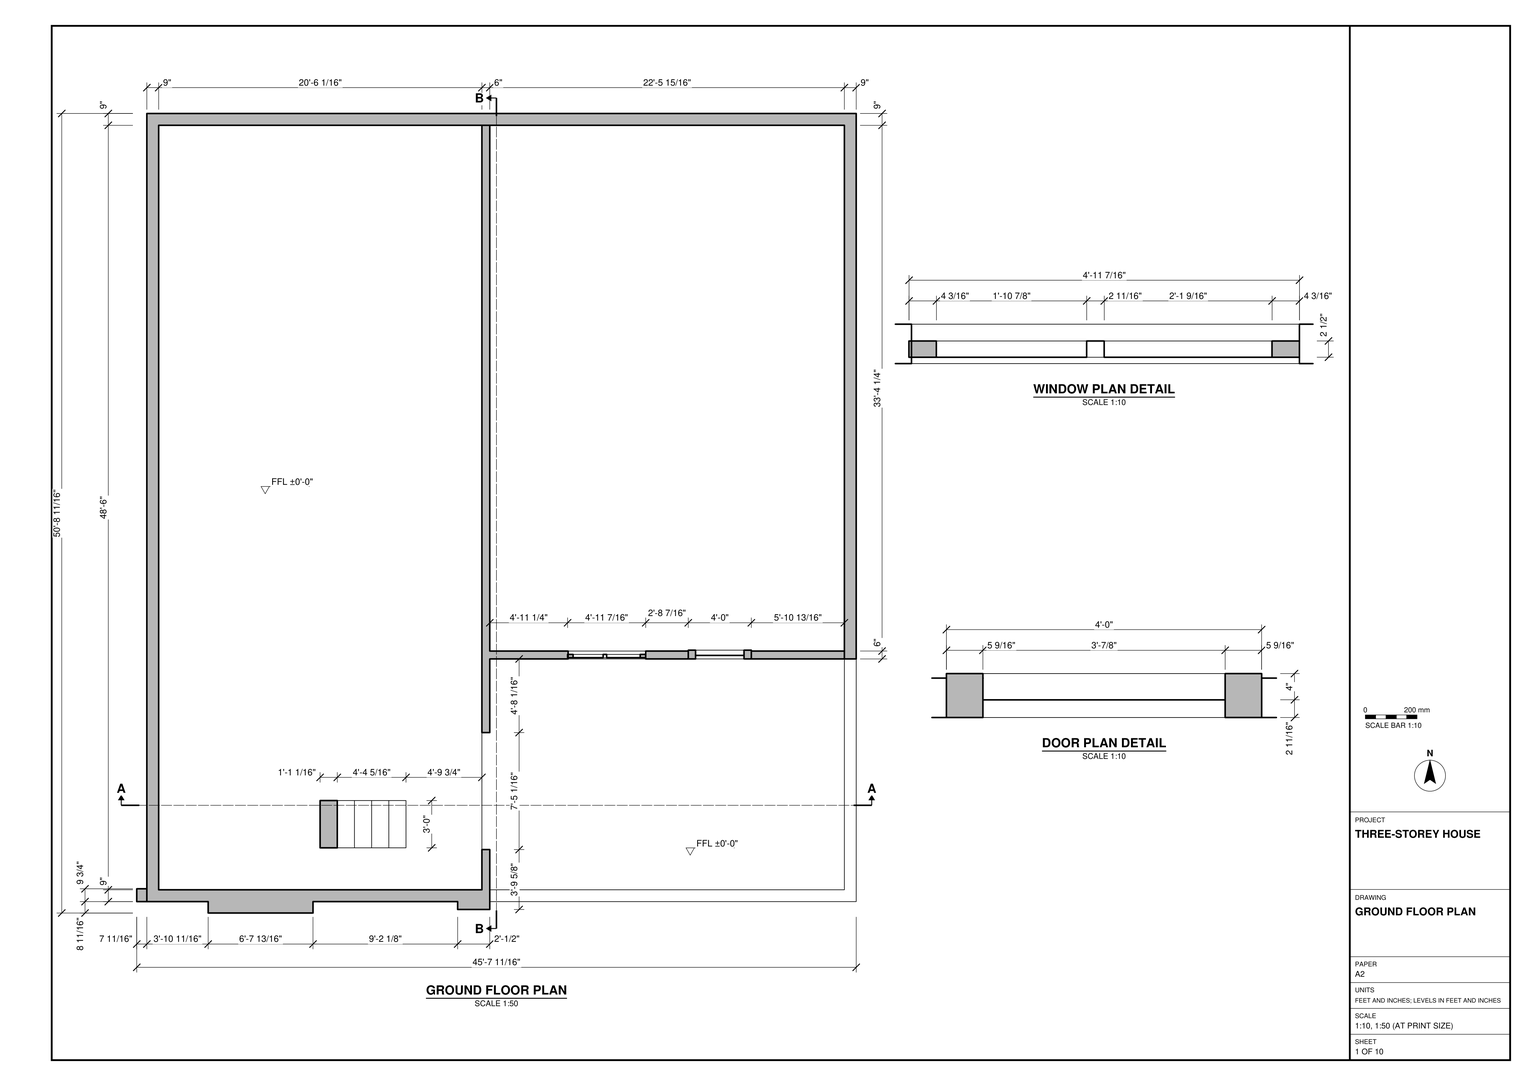
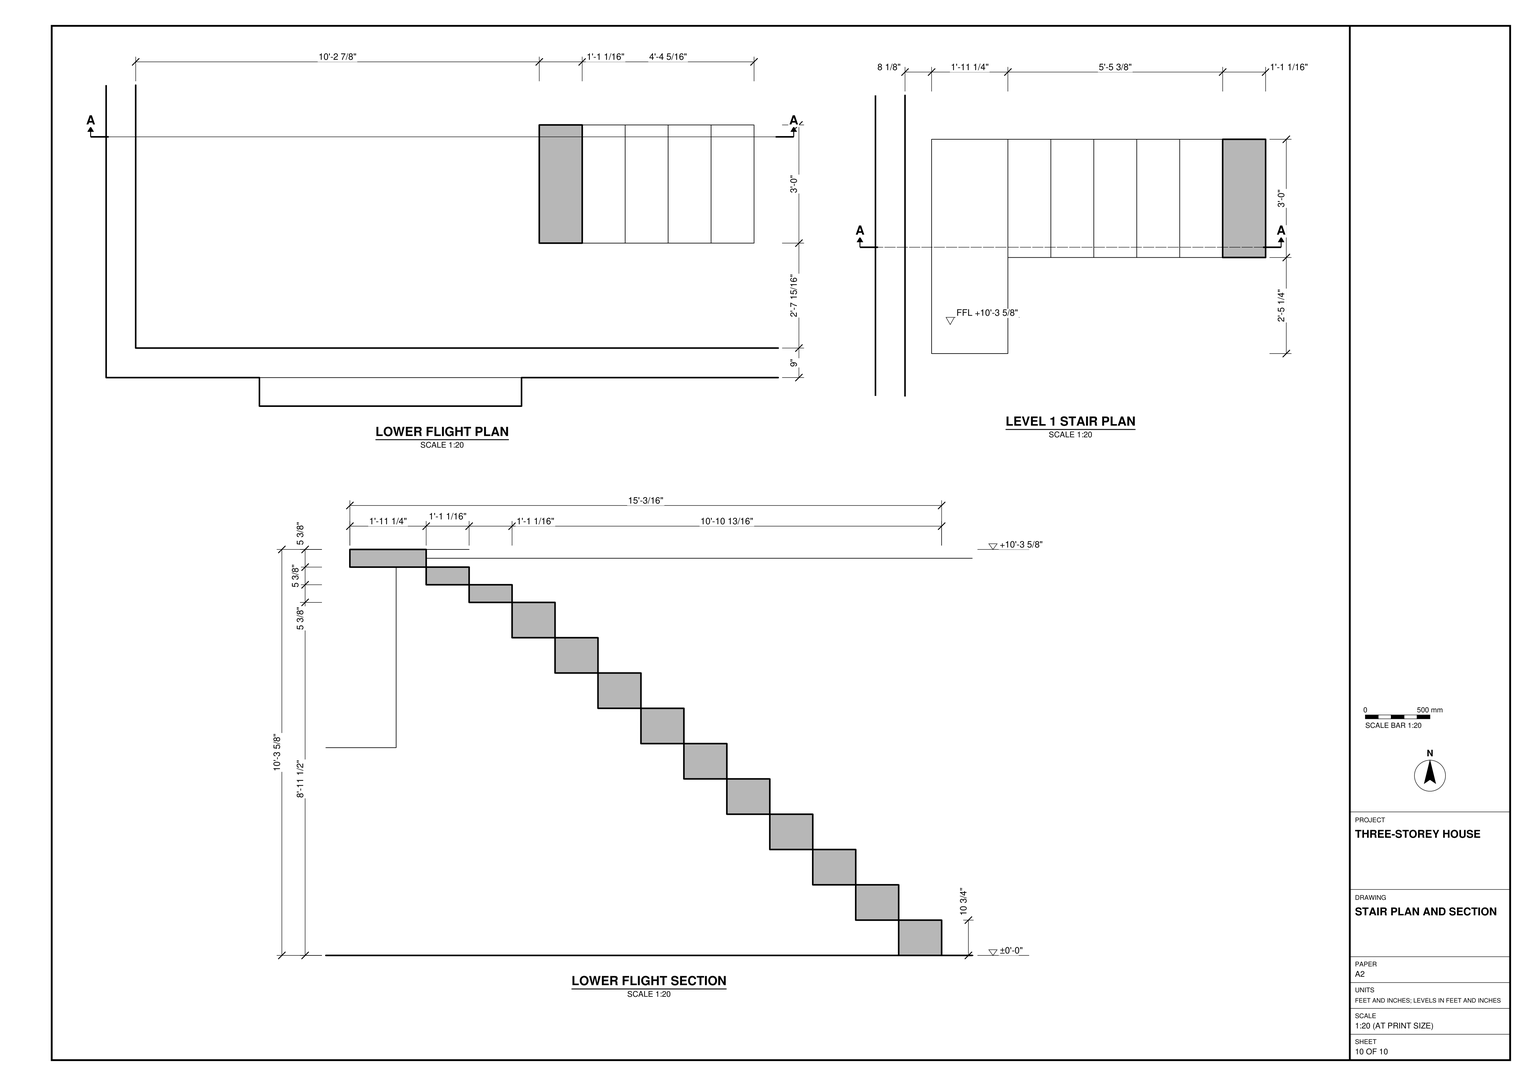
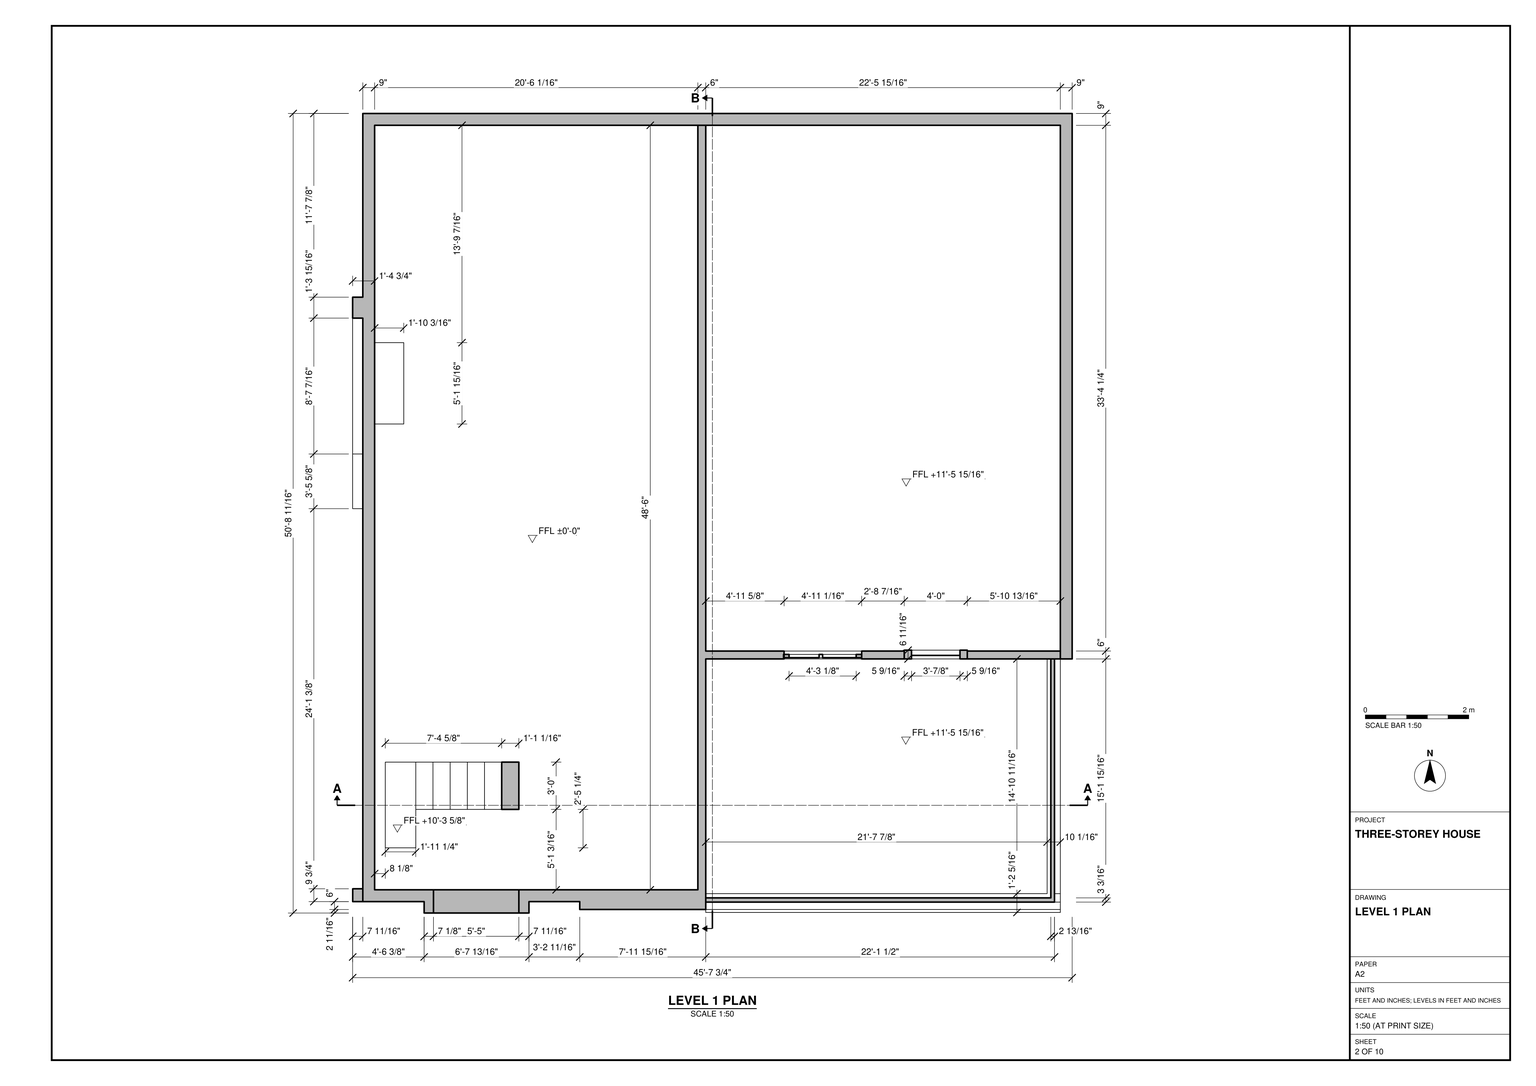
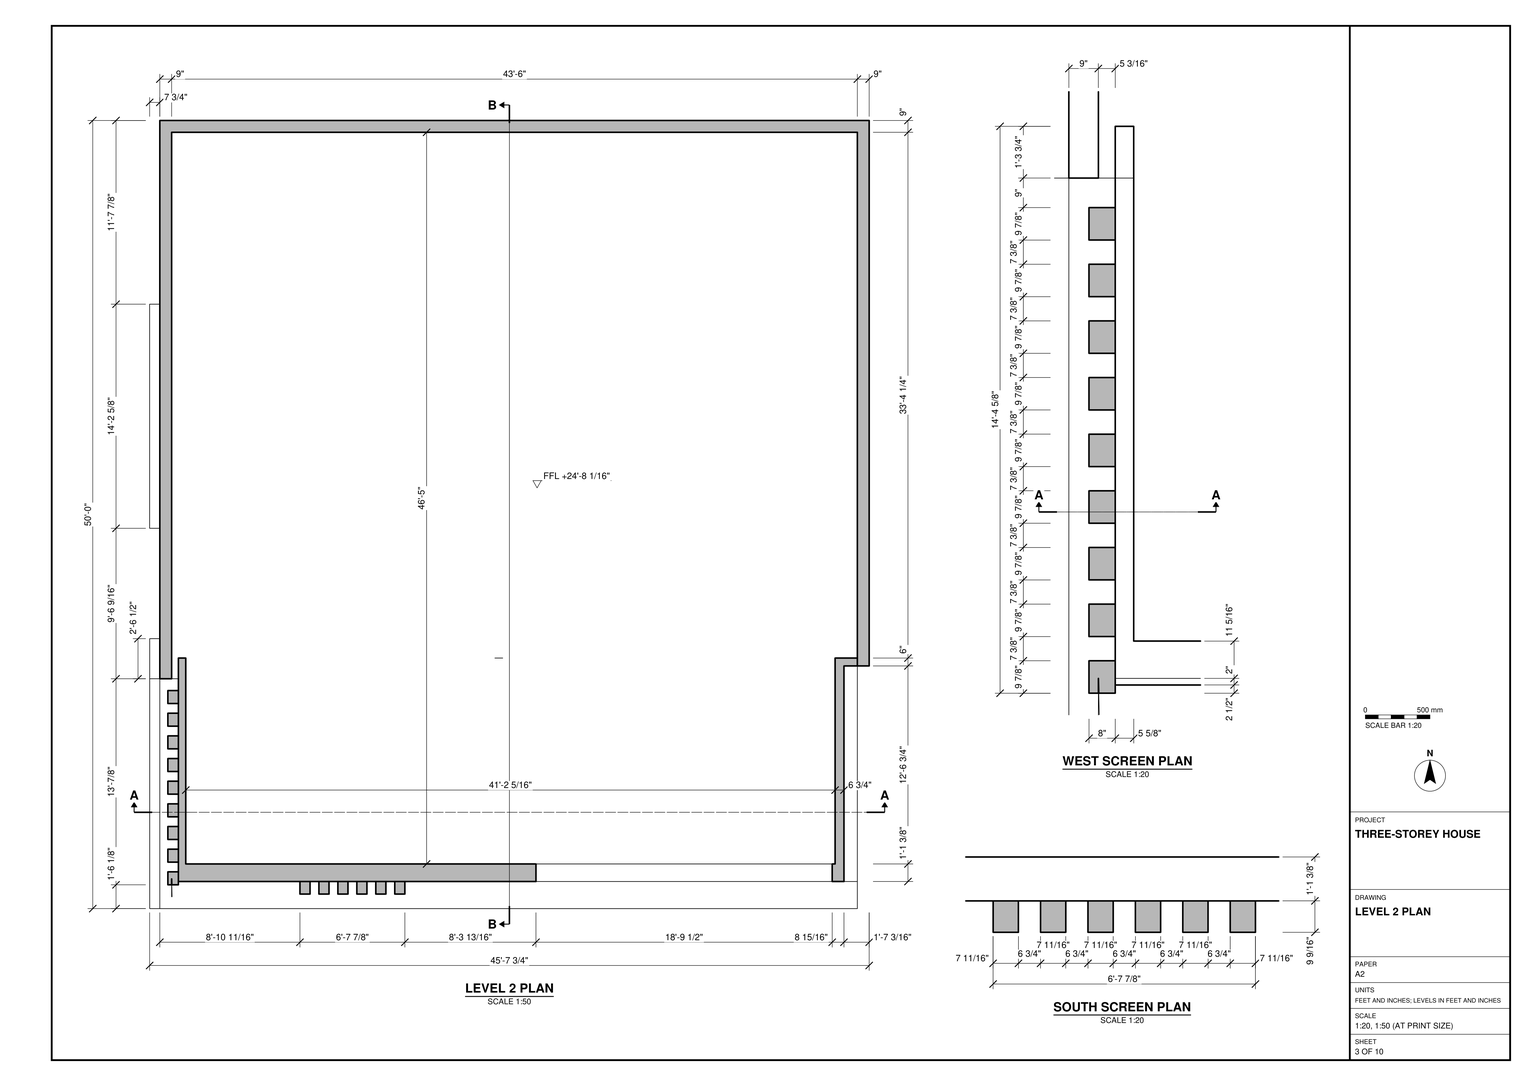
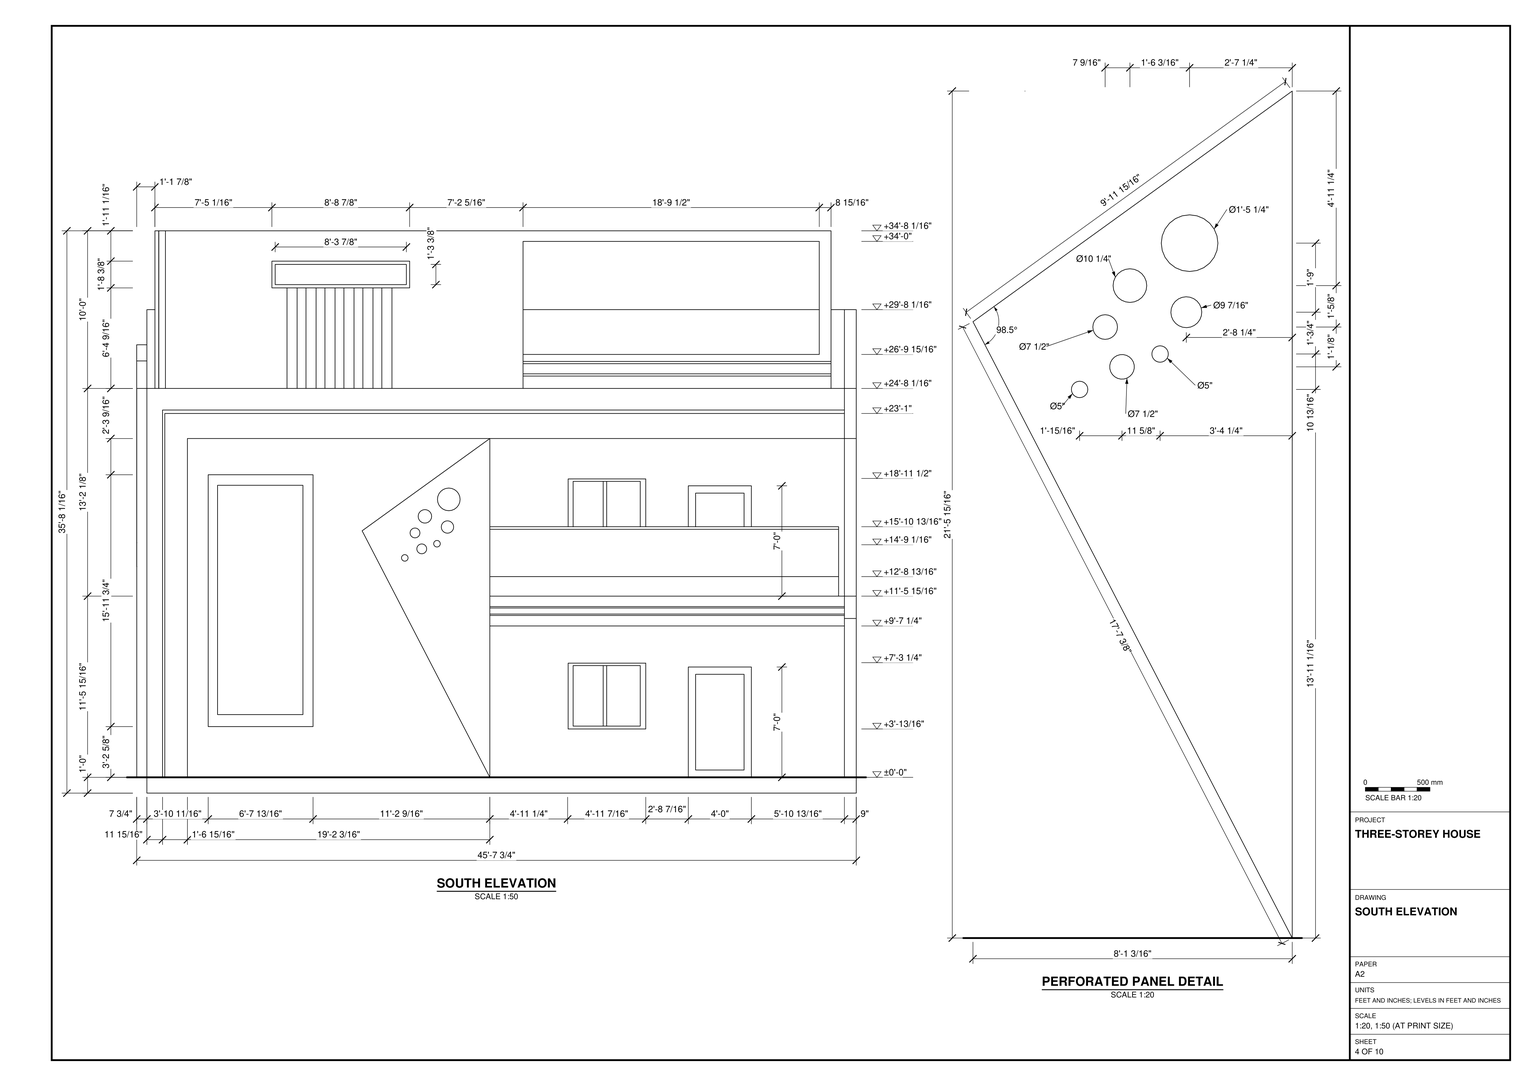
Build the three-storey house in SketchUp from task_files/diagram_01.pdf. Work in feet and inches. Set the overall width to 45'-7 3/4", depth to 50'-8 11/16" and height to 35'-8 1/16". Use finished floor levels of ±0'-0", +11'-5 15/16" and +24'-8 1/16".

Lay out the long west bay beside the wider east bay. Reproduce the wall thicknesses as dimensioned, including the 9" perimeter walls and the 6" dividing wall. Set back the south wall of the enclosed east bay and place its framed window and door according to the plan details. Model the floor slabs at their drawn extents: the Level 1 plan looks down into the west bay, while the east slab continues south beyond the recessed wall. Use the stair plans and section together to place the lower flight, form the individual steps and position the offset landing. Follow the remaining sheets for the upper storey, openings and roof profile. Include built-in joinery and main furniture where shown.

Keep walls, slabs and roof elements in separate groups or components. Group each furniture or joinery piece separately and use components for repeated parts. Any decor or loose items shown may use suitable library components. Save one SketchUp model as output_files/three_storey_house_with_a_recessed_east_bay.skp.

# SketchUp Ruby script. Lengths in inches.
U = 1.inch
M = Sketchup.active_model
def pt(a) = Geom::Point3d.new(a.map { |v| v * U })
def face(e, loops, mat)
  f = e.add_face(loops[0].map { |a| pt(a) })
  loops[1..].each { |l| e.add_face(l.map { |a| pt(a) }).erase! }
  f.material = f.back_material = mat if mat
  f
end
# faces: each face lists its corners as indices into pts; further lists are holes
def faces(e, pts, list, mat = nil) = list.each { |f| face(e, (f[0].is_a?(Array) ? f : [f]).map { |l| l.map { |i| pts[i] } }, mat) }
# xy, xz, yz: faces in a plane at the given z, y or x. An outline is a flat list of corners, or four numbers for a rectangle; further outlines are holes
def ring(l) = l.size == 4 ? [[l[0], l[1]], [l[2], l[1]], [l[2], l[3]], [l[0], l[3]]] : l.each_slice(2).to_a
def flat(e, list, mat, &to3) = list.each { |f| face(e, (f[0].is_a?(Array) ? f : [f]).map { |l| ring(l).map { |u, v| to3.(u, v) } }, mat) }
def xy(e, z, list, mat = nil) = flat(e, list, mat) { |x, y| [x, y, z] }
def xz(e, y, list, mat = nil) = flat(e, list, mat) { |x, z| [x, y, z] }
def yz(e, x, list, mat = nil) = flat(e, list, mat) { |y, z| [x, y, z] }
def lines(e, pts, list) = list.each { |a, b| e.add_line(pt(pts[a]), pt(pts[b])) }
# prism: a flat outline (further loops are holes) pulled along v
def prism(e, loops, v, mat = nil)
  f = face(e, loops, mat); d = Geom::Vector3d.new(v.map { |x| x * U })
  f.pushpull(f.normal.samedirection?(d) ? d.length : -d.length)
end
def box(e, o, s, mat = nil) = prism(e, [[o, [o[0] + s[0], o[1], o[2]], [o[0] + s[0], o[1] + s[1], o[2]], [o[0], o[1] + s[1], o[2]]]], [0, 0, s[2]], mat)
def at(x, y, z, deg = 0) = Geom::Transformation.translation(pt([x, y, z])) * Geom::Transformation.rotation(ORIGIN, Z_AXIS, deg.degrees)
def axes(o, x, y, z) = Geom::Transformation.new([*x, 0, *y, 0, *z, 0, *pt(o).to_a, 1])
def part(name) = M.definitions.add(name)
# library, detail: a bought-in or finely detailed component or shape, given as its bounding box
def library(name, o, s) = part(name).tap { |d| box(d.entities, o, s) }
def detail(e, o, s) = box(e.add_group.entities, o, s)
def put(e, d, t, mat = nil) = e.add_instance(d, t).tap { |i| i.material = mat if mat }
def group(e, t, mat = nil) = e.add_group.tap { |g| g.transformation = t; g.material = mat if mat }.entities
root = M.entities
M.materials.add("[Color A08]").color = [76, 0, 0]
M.materials.add("[Color D05]").color = [255, 191, 0]
M.materials.add("[Color D06]").color = [204, 153, 0]
M.materials.add("[Color E01]").color = [255, 255, 204]
M.materials.add("[Color M05]").color = [114, 114, 114]
M.materials.add("[Color M06]").color = [86, 86, 86]
M.materials.add("[Concrete Form 4x8]").color = [167, 170, 168]
M.materials.add("[Granite Tile]").color = [155, 148, 143]
M.materials.add("[Metal Seamed]").color = [118, 119, 115]
M.materials.add("[Pavers Flagstone Gray]").color = [162, 162, 162]
M.materials.add("[Stone Vein Gray]").color = [166, 165, 165]
M.materials.add("[Translucent Glass Blue]").color = [100, 149, 237]
M.materials["[Translucent Glass Blue]"].alpha = 0.5
M.materials.add("[Translucent Glass Gold]").color = [255, 254, 26]
M.materials["[Translucent Glass Gold]"].alpha = 0.6
M.materials.add("[Translucent Glass Gray]").color = [128, 128, 128]
M.materials["[Translucent Glass Gray]"].alpha = 0.5
c1 = part("Group\#1")
box(c1.entities,[0,0,0],[36,12,3.9375])
c2 = part("Group\#2")
box(c2.entities,[0,0,0],[36,12,3.9375])
c3 = part("Group\#4")
put(c3.entities,c1,at(12,0,82.6875,90))
put(c3.entities,c1,at(24,0,78.75,90))
g1 = group(c3.entities,at(144,0,0))
put(g1,c2,axes([-60,0,39.375],[0,1,0],[-1,0,0],[0,0,2]))
put(g1,c2,axes([-72,0,47.25],[0,1,0],[-1,0,0],[0,0,2]))
put(g1,c2,axes([-96,0,63],[0,1,0],[-1,0,0],[0,0,2]))
put(g1,c2,axes([-108,0,70.875],[0,1,0],[-1,0,0],[0,0,2]))
put(g1,c2,axes([-12,0,7.875],[0,1,0],[-1,0,0],[0,0,2]))
put(g1,c2,axes([-84,0,55.125],[0,1,0],[-1,0,0],[0,0,2]))
put(g1,c2,axes([-48,0,31.5],[0,1,0],[-1,0,0],[0,0,2]))
put(g1,c1,axes([0,0,0],[0,1,0],[-1,0,0],[0,0,2]))
put(g1,c2,axes([-24,0,15.75],[0,1,0],[-1,0,0],[0,0,2]))
put(g1,c2,axes([-36,0,23.625],[0,1,0],[-1,0,0],[0,0,2]))
c4 = part("Group\#7")
xy(c4.entities,0,[[0,0,3.44,17.08]],"[Color A08]")
xy(c4.entities,1.2,[[0,1.2,3.44,8.54],[0,8.54,3.44,9.31],[0,9.31,3.44,15.88]],"[Color A08]")
xy(c4.entities,26.4375,[[0,1.2,3.44,8.54],[0,8.54,3.44,9.31],[0,9.31,3.44,15.88]],"[Color A08]")
xy(c4.entities,27.64,[[0,0,3.44,17.08]],"[Color A08]")
xz(c4.entities,0,[[0,0,3.44,27.64]],"[Color A08]")
xz(c4.entities,1.2,[[0,1.2,3.44,26.4375]],"[Color A08]")
xz(c4.entities,8.54,[[0,1.2,3.44,26.4375]],"[Color A08]")
xz(c4.entities,9.31,[[0,1.2,3.44,26.4375]],"[Color A08]")
xz(c4.entities,15.88,[[0,1.2,3.44,26.4375]],"[Color A08]")
xz(c4.entities,17.08,[[0,0,3.44,27.64]],"[Color A08]")
yz(c4.entities,0,[[[0,0,17.08,27.64],[1.2,1.2,15.88,26.4375]]],"[Color A08]")
yz(c4.entities,0,[[1.2,1.2,8.54,26.4375],[9.31,1.2,15.88,26.4375]],"[Translucent Glass Blue]")
yz(c4.entities,3.44,[[[0,0,17.08,27.64],[1.2,1.2,15.88,26.4375]],[8.54,1.2,9.31,26.4375]],"[Color A08]")
c5 = part("Group\#8")
xy(c5.entities,0,[[0,0,48,6.6875]])
xy(c5.entities,5.56,[[5.56,0,42.44,2.6875],[5.56,2.6875,42.44,6.6875]],"[Color A08]")
xy(c5.entities,78.44,[[5.56,2.6875,42.44,6.6875]])
xy(c5.entities,78.44,[[5.56,0,42.44,2.6875]],"[Color A08]")
xy(c5.entities,84,[[0,0,48,6.6875]],"[Color A08]")
xz(c5.entities,0,[[[0,0,48,84],[5.56,5.56,42.44,78.44]]],"[Color A08]")
xz(c5.entities,2.6875,[[5.56,5.56,42.44,78.44]],"[Color A08]")
xz(c5.entities,6.6875,[[[0,0,48,84],[5.56,5.56,42.44,78.44]]],"[Color A08]")
yz(c5.entities,0,[[0,0,6.6875,84]])
yz(c5.entities,5.56,[[0,5.56,2.6875,78.44],[2.6875,5.56,6.6875,78.44]],"[Color A08]")
yz(c5.entities,42.44,[[2.6875,5.56,6.6875,78.44]])
yz(c5.entities,42.44,[[0,5.56,2.6875,78.44]],"[Color A08]")
yz(c5.entities,48,[[0,0,6.6875,84]],"[Color A08]")
xy(root,0,[[7.75,8.6875,547.75,608.6875]])
xy(root,12,[[7.75,8.6875,7.75,608.6875,547.75,608.6875,547.75,193.4375,538.75,193.4375,538.75,599.6875,16.75,599.6875,16.75,17.6875,262.8125,17.6875,262.8125,48.3125,268.8125,48.3125,268.8125,8.6875],[268.8125,8.6875,547.75,8.6875,547.75,193.4375,538.75,193.4375,538.75,17.6875,268.8125,17.6875],[16.75,17.6875,262.8125,599.6875],[262.8125,137.375,262.8125,599.6875,268.8125,599.6875,268.8125,199.4375,419.92,199.4375,419.92,193.4375,268.8125,193.4375,268.8125,137.375],[467.92,193.4375,538.75,199.4375],
  [268.8125,199.4375,538.75,599.6875]])
xy(root,12,[[0.0625,8.6875,7.75,18.46]],"[Color M05]")
xy(root,12,[[268.8125,17.6875,538.75,17.6875,538.75,193.4375,467.92,193.4375,467.92,199.4375,419.92,199.4375,419.92,193.4375,268.8125,193.4375,268.8125,137.375,262.8125,137.375,262.8125,48.3125,268.8125,48.3125]],"[Concrete Form 4x8]")
xy(root,48.8125,[[328.44,193.4375,387.5,199.4375]])
xy(root,50.625,[[54.43,0,134.24,8.6875]],"[Color M05]")
xy(root,59.76,[[61.55,0,126.55,17.6875]],"[Color M05]")
xy(root,75.27,[[7.75,372.29,38.9375,434.23]])
xy(root,96,[[419.92,193.4375,467.92,199.4375]])
xy(root,98.9375,[[328.44,193.4375,387.5,199.4375]])
xy(root,106.4,[[7.75,269.27,16.75,315.14]])
xy(root,118.63,[[61.55,6.1,126.55,13.16]],"[Color M05]")
xy(root,125.7,[[61.55,6.1,126.55,13.16]],"[Color M05]")
xy(root,127.25,[[268.8125,2.6875,538.75,193.4375]],"[Color E01]")
xy(root,132.9375,[[262.8125,48.3125,268.8125,137.375],[262.8125,137.375,262.8125,599.6875,268.8125,599.6875,268.8125,199.4375,538.75,199.4375,538.75,193.4375,268.8125,193.4375,268.8125,137.375]])
xy(root,135.24,[[268.8125,0.4375,538.75,2.6875]],"[Color D05]")
xy(root,136.3,[[268.8125,0.4375,538.75,2.6875]],"[Color D05]")
xy(root,140.92,[[268.8125,0.4375,538.75,2.6875]],"[Color D05]")
xy(root,141.99,[[268.8125,0.4375,538.75,2.6875]],"[Color D05]")
xy(root,149.9375,[[268.8125,2.6875,538.75,8.3125],[268.8125,8.3125,268.8125,14.75,528.7,14.75,528.7,193.4375,534.3125,193.4375,534.3125,8.3125],[534.3125,8.3125,538.75,14.75],[534.3125,14.75,538.75,193.4375],[419.92,193.4375,467.92,199.4375],
  [467.92,193.4375,538.75,199.4375],[268.8125,199.4375,538.75,599.6875]])
xy(root,149.9375,[[268.8125,14.75,528.7,193.4375]],"[Concrete Form 4x8]")
xy(root,162.02,[[7.75,269.27,16.75,315.14]])
xy(root,164.8125,[[268.8125,8.3125,268.8125,11.53,531.51,11.53,531.51,193.4375,534.3125,193.4375,534.3125,8.3125],[268.8125,11.53,531.51,11.53,531.51,193.4375,528.7,193.4375,528.7,14.75,268.8125,14.75]])
xy(root,165.39,[[7.75,372.29,38.9375,434.23]])
xy(root,172.42,[[0,307.84,7.75,468.84]],"[Color M06]")
xy(root,182.69,[[61.55,4.7,127.8,11.77]],"[Color M05]")
xy(root,189.0625,[[328.44,193.4375,387.5,199.4375]])
xy(root,189.75,[[61.55,4.7,127.8,11.77]],"[Color M05]")
xy(root,190.6,[[0,307.84,7.75,349.46],[0,349.46,7.75,452.89]],"[Color M06]")
xy(root,200.8125,[[268.8125,8.3125,268.8125,11.53,531.51,11.53,531.51,193.4375,534.3125,193.4375,534.3125,8.3125]])
xy(root,202.8125,[[268.8125,8.3125,534.3125,8.3125,534.3125,193.4375,531.51,193.4375,531.51,11.53,268.8125,11.53]],"[Metal Seamed]")
xy(root,204.21,[[7.75,514.29,46.5,576.23]])
xy(root,217.35,[[7.75,372.16,16.75,441.53]])
xy(root,233.9375,[[419.92,193.4375,467.92,199.4375]])
xy(root,234.33,[[61.55,0,126.55,17.6875]],"[Color M05]")
xy(root,239.1875,[[328.44,193.4375,387.5,199.4375]])
xy(root,242.375,[[54.43,0,134.24,8.6875]],"[Color M05]")
xy(root,257.21,[[7.75,269.27,187.4375,315.14]])
xy(root,269.9375,[[268.8125,8.6875,538.75,193.4375]])
xy(root,294.34,[[7.75,514.29,46.5,576.23]])
xy(root,300.5,[[0.0625,18.46,7.75,214.2]],"[Color M05]")
xy(root,302.0625,[[27.5,42.6875,27.5,183.68,16.75,183.68,16.75,599.6875,538.75,599.6875,538.75,199.4375,521.8125,199.4375,521.8125,42.6875]])
xy(root,304.27,[[7.75,269.27,187.4375,315.14]])
xy(root,308.0625,[[7.75,8.6875,538.75,8.6875,538.75,29.3125,194.3,29.3125,194.3,19.75,186.61,19.75,186.61,29.3125,179.86,29.3125,179.86,19.75,172.17,19.75,172.17,29.3125,165.42,29.3125,165.42,19.75,157.73,19.75,157.73,29.3125,150.98,29.3125,150.98,19.75,143.3,19.75,143.3,29.3125,136.55,29.3125,136.55,19.75,128.86,19.75,128.86,29.3125,122.11,29.3125,122.11,19.75,114.42,19.75,114.42,29.3125,21.875,29.3125,21.875,26.82,16.85,26.82,17.06,17.6875,16.75,17.6875,16.75,26.82,13.875,26.82,13.875,36.69,21.875,36.69,21.875,44.07,13.875,44.07,13.875,53.94,21.875,53.94,21.875,61.32,13.875,61.32,13.875,71.19,21.875,71.19,21.875,78.57,13.875,78.57,13.875,88.44,21.875,88.44,21.875,95.82,13.875,95.82,13.875,105.69,21.875,105.69,21.875,113.07,13.875,113.07,13.875,122.94,21.875,122.94,21.875,130.32,13.875,130.32,13.875,140.19,21.875,140.19,21.875,147.57,13.875,147.57,13.875,157.44,21.875,157.44,21.875,164.82,13.875,164.82,13.875,174.69,21.875,174.69,21.875,183.68,7.75,183.68],[16.75,17.6875,17.06,17.6875,16.85,26.82,16.75,26.82],[114.42,19.75,122.11,29.3125],[128.86,19.75,136.55,29.3125],[143.3,19.75,150.98,29.3125],
  [157.73,19.75,165.42,29.3125],[172.17,19.75,179.86,29.3125],[186.61,19.75,194.3,29.3125],[16.75,26.82,16.85,26.82,16.75,31.32],[21.875,29.3125,48.69,31.32],
  [48.69,29.3125,262.8125,42.6875],[262.8125,29.3125,262.8125,42.6875,521.8125,42.6875,521.8125,199.4375,538.75,199.4375,538.75,193.4375,528.5625,193.4375,528.5625,29.3125],[528.5625,29.3125,538.75,193.4375],[21.875,31.32,48.69,31.32,48.69,42.6875,27.5,42.6875,27.5,183.68,21.875,183.68],[27.5,42.6875,521.8125,42.6875,521.8125,199.4375,538.75,199.4375,538.75,599.6875,16.75,599.6875,16.75,183.68,21.875,183.68,21.875,199.4375,27.5,199.4375],
  [21.875,183.68,27.5,199.4375]])
xy(root,308.0625,[[0.0625,8.6875,7.75,183.68],[0.0625,183.68,7.75,214.2]],"[Color M05]")
xy(root,323.66,[[7.75,372.16,16.75,441.53]])
xy(root,329.01,[[0,298.21,7.75,349.46],[0,349.46,7.75,452.89]],"[Color M06]")
xy(root,333.96,[[294.1,29.3125,519.6,42.6875]])
xy(root,341.32,[[0,298.21,7.75,468.84]],"[Color M06]")
xy(root,368.0625,[[7.75,183.68,16.75,183.68,16.75,599.6875,538.75,599.6875,538.75,193.4375,547.75,193.4375,547.75,608.6875,7.75,608.6875],[528.5625,193.4375,538.75,199.4375]])
xy(root,384.62,[[114.42,25.625,122.11,29.3125],[128.86,25.625,136.55,29.3125],[143.3,25.625,150.98,29.3125],[157.73,25.625,165.42,29.3125],[172.17,25.625,179.86,29.3125],
  [186.61,25.625,194.3,29.3125]])
xy(root,384.62,[[114.42,19.75,122.11,25.625],[128.86,19.75,136.55,25.625],[143.3,19.75,150.98,25.625],[157.73,19.75,165.42,25.625],[172.17,19.75,179.86,25.625],
  [186.61,19.75,194.3,25.625],[102.92,25.625,114.42,29.3125],[122.11,25.625,128.86,29.3125],[136.55,25.625,143.3,29.3125],[150.98,25.625,157.73,29.3125],
  [165.42,25.625,172.17,29.3125],[179.86,25.625,186.61,29.3125],[194.3,25.625,207.78,29.3125]],"[Color M05]")
xy(root,387.11,[[105.41,29.3125,205.29,42.6875]])
xy(root,387.11,[[105.41,25.625,205.29,29.3125]],"[Color M05]")
xy(root,402.49,[[105.41,29.3125,205.29,42.6875]])
xy(root,402.49,[[105.41,25.625,205.29,29.3125]],"[Color M05]")
xy(root,404.98,[[102.92,25.625,207.78,29.3125]],"[Color M05]")
xy(root,420.02,[[294.1,29.3125,519.6,42.6875]])
xy(root,422.0625,[[[27.5,42.6875,521.8125,199.4375],[311.79,85.54,329.04,164.1],[348.29,85.54,365.54,164.1],[384.79,85.54,402.04,164.1],[421.29,85.54,438.54,164.1],[457.79,85.54,475.04,164.1],[494.29,85.54,511.54,164.1]]])
xy(root,428.0625,[[21.875,29.3125,528.5625,29.3125,528.5625,42.6875,27.5,42.6875,27.5,199.4375,21.875,199.4375],[[27.5,42.6875,521.8125,199.4375],[311.79,85.54,329.04,164.1],[348.29,85.54,365.54,164.1],[384.79,85.54,402.04,164.1],[421.29,85.54,438.54,164.1],[457.79,85.54,475.04,164.1],[494.29,85.54,511.54,164.1]],[521.8125,42.6875,528.5625,199.4375]])
xy(root,428.0625,[[13.875,26.82,16.75,26.82,16.75,31.32,16.85,26.82,21.875,26.82,21.875,36.69,13.875,36.69],[13.875,44.07,21.875,53.94],[13.875,61.32,21.875,71.19],[13.875,78.57,21.875,88.44],[13.875,95.82,21.875,105.69],
  [13.875,113.07,21.875,122.94],[13.875,130.32,21.875,140.19],[13.875,147.57,21.875,157.44],[13.875,164.82,21.875,174.69]],"[Color M05]")
xz(root,0,[[[54.43,50.625,134.24,242.375],[61.55,59.76,126.55,234.33]]],"[Color M05]")
xz(root,0,[[61.55,59.76,126.55,234.33]],"[Translucent Glass Blue]")
xz(root,0.4375,[[268.8125,135.24,538.75,136.3],[268.8125,140.92,538.75,141.99]],"[Color D05]")
xz(root,2.6875,[[268.8125,127.25,538.75,135.24],[268.8125,136.3,538.75,140.92],[268.8125,141.99,538.75,149.9375]])
xz(root,2.6875,[[204.07,176.57,204.72,176.65,205.32,176.9,205.84,177.3,206.23,177.82,206.48,178.42,206.57,179.07,206.48,179.72,206.23,180.32,205.84,180.84,205.32,181.23,204.72,181.48,204.07,181.57,203.42,181.48,202.82,181.23,202.3,180.84,201.9,180.32,201.65,179.72,201.57,179.07,201.65,178.42,201.9,177.82,202.3,177.3,202.82,176.9,203.42,176.65],[216.57,182.22,217.55,182.24,218.49,182.52,219.33,183.02,220.01,183.73,220.48,184.59,220.71,185.54,220.6875,186.52,220.42,187.46,219.91,188.3,219.2,188.97,218.34,189.44,217.39,189.68,216.41,189.66,215.47,189.38,214.64,188.875,213.96,188.17,213.49,187.31,213.25,186.36,213.28,185.38,213.55,184.44,214.06,183.6,214.76,182.93,215.62,182.45],[228.58,187.36,229.23,187.44,229.83,187.69,230.35,188.09,230.74,188.61,230.99,189.21,231.08,189.86,230.99,190.51,230.74,191.11,230.35,191.625,229.83,192.02,229.23,192.27,228.58,192.36,227.93,192.27,227.33,192.02,226.81,191.625,226.41,191.11,226.16,190.51,226.08,189.86,226.16,189.21,226.41,188.61,226.81,188.09,227.33,187.69,227.93,187.44],[211.84,194.32,212.81,194.45,213.72,194.82,214.5,195.42,215.09,196.19,215.47,197.1,215.6,198.07,215.47,199.04,215.1,199.94,214.5,200.72,213.72,201.32,212.82,201.69,211.85,201.82,210.88,201.69,209.97,201.32,209.2,200.72,208.6,199.95,208.22,199.04,208.1,198.07,208.22,197.1,208.6,196.2,209.19,195.42,209.97,194.82,210.875,194.45],[236.67,197.88,237.88,198.07,239.01,198.57,239.96,199.34,240.6875,200.33,241.13,201.47,241.27,202.69,241.08,203.91,240.58,205.03,239.8125,205.99,238.82,206.71,237.68,207.16,236.46,207.29,235.24,207.1,234.12,206.6,233.16,205.84,232.4375,204.84,231.99,203.7,231.86,202.48,232.05,201.27,232.54,200.14,233.3125,199.18,234.3,198.46,235.45,198.02],
  [219.39,205.57,220.72,205.74,221.95,206.25,223.01,207.07,223.83,208.13,224.34,209.36,224.51,210.69,224.34,212.02,223.83,213.25,223.01,214.31,221.95,215.13,220.72,215.64,219.39,215.82,218.0625,215.64,216.83,215.13,215.76,214.31,214.95,213.25,214.4375,212.02,214.26,210.69,214.4375,209.36,214.95,208.13,215.76,207.07,216.83,206.25,218.0625,205.74],[237.56,214.99,239.79,215.28,241.87,216.14,243.66,217.51,245.03,219.3,245.89,221.38,246.19,223.61,245.89,225.84,245.03,227.92,243.66,229.71,241.87,231.08,239.79,231.94,237.56,232.24,235.33,231.94,233.25,231.08,231.46,229.71,230.09,227.92,229.23,225.84,228.94,223.61,229.23,221.38,230.09,219.3,231.46,217.51,233.25,216.14,235.33,215.28]],"[Color D05]")
xz(root,2.6875,[[[268.8125,12,268.8125,269.9375,171.6,199.69],[237.56,214.99,235.33,215.28,233.25,216.14,231.46,217.51,230.09,219.3,229.23,221.38,228.94,223.61,229.23,225.84,230.09,227.92,231.46,229.71,233.25,231.08,235.33,231.94,237.56,232.24,239.79,231.94,241.87,231.08,243.66,229.71,245.03,227.92,245.89,225.84,246.19,223.61,245.89,221.38,245.03,219.3,243.66,217.51,241.87,216.14,239.79,215.28],[219.39,205.57,218.0625,205.74,216.83,206.25,215.76,207.07,214.95,208.13,214.4375,209.36,214.26,210.69,214.4375,212.02,214.95,213.25,215.76,214.31,216.83,215.13,218.0625,215.64,219.39,215.82,220.72,215.64,221.95,215.13,223.01,214.31,223.83,213.25,224.34,212.02,224.51,210.69,224.34,209.36,223.83,208.13,223.01,207.07,221.95,206.25,220.72,205.74],[236.67,197.88,235.45,198.02,234.3,198.46,233.3125,199.18,232.54,200.14,232.05,201.27,231.86,202.48,231.99,203.7,232.4375,204.84,233.16,205.84,234.12,206.6,235.24,207.1,236.46,207.29,237.68,207.16,238.82,206.71,239.8125,205.99,240.58,205.03,241.08,203.91,241.27,202.69,241.13,201.47,240.6875,200.33,239.96,199.34,239.01,198.57,237.88,198.07],[211.84,194.32,210.875,194.45,209.97,194.82,209.19,195.42,208.6,196.2,208.22,197.1,208.1,198.07,208.22,199.04,208.6,199.95,209.2,200.72,209.97,201.32,210.88,201.69,211.85,201.82,212.82,201.69,213.72,201.32,214.5,200.72,215.1,199.94,215.47,199.04,215.6,198.07,215.47,197.1,215.09,196.19,214.5,195.42,213.72,194.82,212.81,194.45],[216.57,182.22,215.62,182.45,214.76,182.93,214.06,183.6,213.55,184.44,213.28,185.38,213.25,186.36,213.49,187.31,213.96,188.17,214.64,188.875,215.47,189.38,216.41,189.66,217.39,189.68,218.34,189.44,219.2,188.97,219.91,188.3,220.42,187.46,220.6875,186.52,220.71,185.54,220.48,184.59,220.01,183.73,219.33,183.02,218.49,182.52,217.55,182.24],[204.07,176.57,203.42,176.65,202.82,176.9,202.3,177.3,201.9,177.82,201.65,178.42,201.57,179.07,201.65,179.72,201.9,180.32,202.3,180.84,202.82,181.23,203.42,181.48,204.07,181.57,204.72,181.48,205.32,181.23,205.84,180.84,206.23,180.32,206.48,179.72,206.57,179.07,206.48,178.42,206.23,177.82,205.84,177.3,205.32,176.9,204.72,176.65],[228.58,187.36,227.93,187.44,227.33,187.69,226.81,188.09,226.41,188.61,226.16,189.21,226.08,189.86,226.16,190.51,226.41,191.11,226.81,191.625,227.33,192.02,227.93,192.27,228.58,192.36,229.23,192.27,229.83,192.02,230.35,191.625,230.74,191.11,230.99,190.51,231.08,189.86,230.99,189.21,230.74,188.61,230.35,188.09,229.83,187.69,229.23,187.44]]],"[Color M05]")
xz(root,4.7,[[61.55,182.69,127.8,189.75]],"[Color M05]")
xz(root,6.1,[[61.55,118.63,126.55,125.7]],"[Color M05]")
xz(root,8.3125,[[268.8125,149.9375,534.3125,164.8125]])
xz(root,8.3125,[[268.8125,200.8125,534.3125,202.8125]],"[Metal Seamed]")
xz(root,8.3125,[[268.8125,164.8125,534.3125,200.8125]],"[Translucent Glass Blue]")
xz(root,8.6875,[[19.67,12,21.38,12,21.38,289,538.75,289,538.75,291.625,19.67,291.625]])
xz(root,8.6875,[[0.0625,12,7.75,308.0625],[7.75,12,19.67,12,19.67,291.625,538.75,291.625,538.75,308.0625,7.75,308.0625],[21.38,12,38.61,12,38.61,269.9375,538.75,269.9375,538.75,289,21.38,289]],"[Color M05]")
xz(root,8.6875,[[7.75,0,547.75,12]],"[Granite Tile]")
xz(root,8.6875,[[[38.61,12,268.8125,12,171.6,199.69,268.8125,269.9375,38.61,269.9375],[54.43,50.625,134.24,242.375]]],"[Pavers Flagstone Gray]")
xz(root,11.53,[[268.8125,200.8125,531.51,202.8125]],"[Metal Seamed]")
xz(root,11.53,[[268.8125,164.8125,531.51,200.8125]],"[Translucent Glass Blue]")
xz(root,11.77,[[61.55,182.69,127.8,189.75]])
xz(root,13.16,[[61.55,118.63,126.55,125.7]])
xz(root,14.75,[[268.8125,149.9375,528.7,164.8125]])
xz(root,17.6875,[[[16.75,12,262.8125,269.9375],[61.55,59.76,126.55,234.33]]])
xz(root,17.6875,[[61.55,59.76,126.55,234.33]],"[Translucent Glass Blue]")
xz(root,18.46,[[0.0625,12,7.75,300.5]],"[Color M05]")
xz(root,19.75,[[114.42,308.0625,122.11,384.62],[128.86,308.0625,136.55,384.62],[143.3,308.0625,150.98,384.62],[157.73,308.0625,165.42,384.62],[172.17,308.0625,179.86,384.62],
  [186.61,308.0625,194.3,384.62]],"[Color M05]")
xz(root,25.625,[[[102.92,384.62,207.78,404.98],[105.41,387.11,205.29,402.49]]],"[Color M05]")
xz(root,26.82,[[13.875,308.0625,16.75,428.0625],[16.85,308.0625,21.875,428.0625]],"[Color M05]")
xz(root,29.3125,[[114.42,308.0625,122.11,384.62],[122.11,308.0625,128.86,384.62],[128.86,308.0625,136.55,384.62],[136.55,308.0625,143.3,384.62],[143.3,308.0625,150.98,384.62],
  [150.98,308.0625,157.73,384.62],[157.73,308.0625,165.42,384.62],[165.42,308.0625,172.17,384.62],[172.17,308.0625,179.86,384.62],[179.86,308.0625,186.61,384.62],
  [186.61,308.0625,194.3,384.62],[294.1,308.0625,528.5625,317.48],[294.1,319.18,528.5625,326.92],[[102.92,384.62,207.78,404.98],[105.41,387.11,205.29,402.49]]])
xz(root,29.3125,[[294.1,317.48,528.5625,319.18],[294.1,326.92,528.5625,328.62]],"[Color D05]")
xz(root,29.3125,[[21.875,308.0625,114.42,308.0625,114.42,384.62,102.92,384.62,102.92,404.98,207.78,404.98,207.78,384.62,194.3,384.62,194.3,308.0625,294.1,308.0625,294.1,420.02,519.6,420.02,519.6,333.96,294.1,333.96,294.1,328.62,528.5625,328.62,528.5625,428.0625,21.875,428.0625]],"[Color E01]")
xz(root,36.69,[[13.875,308.0625,21.875,428.0625]],"[Color M05]")
xz(root,42.6875,[[27.5,302.0625,48.69,308.0625],[48.69,302.0625,262.8125,308.0625],[262.8125,302.0625,521.8125,308.0625],[[27.5,308.0625,521.8125,422.0625],[294.1,333.96,519.6,420.02],[105.41,387.11,205.29,402.49]],[27.5,422.0625,521.8125,428.0625]])
xz(root,44.07,[[13.875,308.0625,21.875,428.0625]],"[Color M05]")
xz(root,48.3125,[[262.8125,12,268.8125,132.9375]])
xz(root,53.94,[[13.875,308.0625,21.875,428.0625]],"[Color M05]")
xz(root,61.32,[[13.875,308.0625,21.875,428.0625]],"[Color M05]")
xz(root,71.19,[[13.875,308.0625,21.875,428.0625]],"[Color M05]")
xz(root,78.57,[[13.875,308.0625,21.875,428.0625]],"[Color M05]")
xz(root,85.54,[[311.79,422.0625,329.04,428.0625],[348.29,422.0625,365.54,428.0625],[384.79,422.0625,402.04,428.0625],[421.29,422.0625,438.54,428.0625],[457.79,422.0625,475.04,428.0625],
  [494.29,422.0625,511.54,428.0625]])
xz(root,88.44,[[13.875,308.0625,21.875,428.0625]],"[Color M05]")
xz(root,95.82,[[13.875,308.0625,21.875,428.0625]],"[Color M05]")
xz(root,105.69,[[13.875,308.0625,21.875,428.0625]],"[Color M05]")
xz(root,113.07,[[13.875,308.0625,21.875,428.0625]],"[Color M05]")
xz(root,122.94,[[13.875,308.0625,21.875,428.0625]],"[Color M05]")
xz(root,130.32,[[13.875,308.0625,21.875,428.0625]],"[Color M05]")
xz(root,137.375,[[262.8125,12,268.8125,132.9375]])
xz(root,140.19,[[13.875,308.0625,21.875,428.0625]],"[Color M05]")
xz(root,147.57,[[13.875,308.0625,21.875,428.0625]],"[Color M05]")
xz(root,157.44,[[13.875,308.0625,21.875,428.0625]],"[Color M05]")
xz(root,164.1,[[311.79,422.0625,329.04,428.0625],[348.29,422.0625,365.54,428.0625],[384.79,422.0625,402.04,428.0625],[421.29,422.0625,438.54,428.0625],[457.79,422.0625,475.04,428.0625],
  [494.29,422.0625,511.54,428.0625]])
xz(root,164.82,[[13.875,308.0625,21.875,428.0625]],"[Color M05]")
xz(root,174.69,[[13.875,308.0625,21.875,428.0625]],"[Color M05]")
xz(root,183.68,[[16.75,302.0625,18,308.0625],[18,302.0625,27.5,308.0625],[7.75,308.0625,16.75,368.0625]])
xz(root,193.4375,[[538.75,12,547.75,132.9375],[268.8125,127.25,538.75,132.9375],[268.8125,132.9375,538.75,149.9375],[538.75,132.9375,547.75,149.9375],[538.75,149.9375,547.75,269.9375],
  [531.51,164.8125,534.3125,200.8125],[531.51,200.8125,534.3125,202.8125],[538.75,269.9375,547.75,308.0625],[528.5625,308.0625,538.75,368.0625],[538.75,308.0625,547.75,368.0625]])
xz(root,193.4375,[[[268.8125,12,419.92,12,419.92,96,467.92,96,467.92,12,538.75,12,538.75,127.25,268.8125,127.25],[328.44,48.8125,387.5,98.9375]],[[268.8125,149.9375,419.92,149.9375,419.92,233.9375,467.92,233.9375,467.92,149.9375,528.7,149.9375,528.7,164.8125,531.51,164.8125,531.51,202.8125,534.3125,202.8125,534.3125,149.9375,538.75,149.9375,538.75,269.9375,268.8125,269.9375],[328.44,189.0625,387.5,239.1875]]],"[Color E01]")
xz(root,199.4375,[[[268.8125,12,268.8125,132.9375,538.75,132.9375,538.75,12,467.92,12,467.92,96,419.92,96,419.92,12],[328.44,48.8125,387.5,98.9375]],[268.8125,132.9375,538.75,149.9375],[[268.8125,149.9375,268.8125,269.9375,538.75,269.9375,538.75,149.9375,467.92,149.9375,467.92,233.9375,419.92,233.9375,419.92,149.9375],[328.44,189.0625,387.5,239.1875]],[521.8125,302.0625,538.75,308.0625],[21.875,308.0625,27.5,428.0625],
  [521.8125,308.0625,521.8125,428.0625,528.5625,428.0625,528.5625,368.0625,538.75,368.0625,538.75,308.0625],[27.5,422.0625,521.8125,428.0625]])
xz(root,214.2,[[0.0625,300.5,7.75,308.0625]],"[Color M05]")
xz(root,269.27,[[7.75,106.4,16.75,162.02],[7.75,257.21,187.4375,304.27]])
xz(root,298.21,[[0,329.01,7.75,341.32]],"[Color M06]")
xz(root,307.84,[[0,172.42,7.75,190.6]],"[Color M06]")
xz(root,315.14,[[7.75,106.4,16.75,162.02],[7.75,257.21,187.4375,304.27]])
xz(root,372.16,[[7.75,217.35,16.75,323.66]])
xz(root,372.29,[[7.75,75.27,38.9375,165.39]])
xz(root,434.23,[[7.75,75.27,38.9375,165.39]])
xz(root,441.53,[[7.75,217.35,16.75,323.66]])
xz(root,452.89,[[0,190.6,7.75,329.01]],"[Color M06]")
xz(root,468.84,[[0,172.42,7.75,190.6],[0,190.6,7.75,329.01],[0,329.01,7.75,341.32]],"[Color M06]")
xz(root,514.29,[[7.75,204.21,46.5,294.34]])
xz(root,576.23,[[7.75,204.21,46.5,294.34]])
xz(root,599.6875,[[16.75,12,262.8125,132.9375],[262.8125,12,268.8125,132.9375],[268.8125,12,538.75,132.9375],[16.75,132.9375,262.8125,149.9375],[262.8125,132.9375,268.8125,149.9375],
  [268.8125,132.9375,538.75,149.9375],[16.75,149.9375,262.8125,269.9375],[262.8125,149.9375,268.8125,269.9375],[268.8125,149.9375,538.75,269.9375],[16.75,269.9375,262.8125,302.0625],
  [262.8125,269.9375,268.8125,293.9375],[268.8125,269.9375,538.75,302.0625],[262.8125,293.9375,268.8125,302.0625],[16.75,302.0625,262.8125,308.0625],[262.8125,302.0625,268.8125,308.0625],
  [268.8125,302.0625,538.75,308.0625],[16.75,308.0625,538.75,368.0625]])
xz(root,608.6875,[[7.75,0,547.75,12],[7.75,12,547.75,368.0625]])
yz(root,0,[[307.84,172.42,468.84,190.6],[452.89,190.6,452.89,329.01,298.21,329.01,298.21,341.32,468.84,341.32,468.84,190.6]],"[Color M06]")
yz(root,0.0625,[[8.6875,12,8.6875,308.0625,214.2,308.0625,214.2,300.5,18.46,300.5,18.46,12]],"[Color M05]")
yz(root,7.75,[[8.6875,0,214.2,12],[214.2,0,608.6875,12],[[214.2,12,214.2,368.0625,349.46,368.0625,349.46,341.32,298.21,341.32,298.21,329.01,349.46,329.01,349.46,190.6,307.84,190.6,307.84,172.42,468.84,172.42,468.84,368.0625,608.6875,368.0625,608.6875,12],[514.29,204.21,576.23,294.34],[372.29,75.27,434.23,165.39],[269.27,106.4,315.14,162.02],[269.27,257.21,315.14,304.27]],[183.68,308.0625,214.2,368.0625]])
yz(root,7.75,[[[349.46,190.6,452.89,329.01],[372.16,217.35,441.53,323.66]],[349.46,341.32,468.84,368.0625]],"[Color D06]")
yz(root,7.75,[[8.6875,12,18.46,12,18.46,300.5,214.2,300.5,214.2,308.0625,8.6875,308.0625],[18.46,12,214.2,300.5]],"[Color M05]")
yz(root,13.875,[[26.82,308.0625,36.69,428.0625],[44.07,308.0625,53.94,428.0625],[61.32,308.0625,71.19,428.0625],[78.57,308.0625,88.44,428.0625],[95.82,308.0625,105.69,428.0625],
  [113.07,308.0625,122.94,428.0625],[130.32,308.0625,140.19,428.0625],[147.57,308.0625,157.44,428.0625],[164.82,308.0625,174.69,428.0625]],"[Color M05]")
yz(root,16.75,[[269.27,106.4,315.14,132.9375],[17.6875,132.9375,269.27,149.9375],[269.27,132.9375,315.14,149.9375],[315.14,132.9375,599.6875,149.9375],[17.6875,149.9375,269.27,149.9375,269.27,162.02,315.14,162.02,315.14,149.9375,599.6875,149.9375,599.6875,269.9375,441.53,269.9375,441.53,217.35,372.16,217.35,372.16,269.9375,17.6875,269.9375],
  [269.27,149.9375,315.14,162.02],[372.16,217.35,441.53,269.9375],[372.16,269.9375,441.53,302.0625],[183.68,302.0625,372.16,308.0625],[372.16,302.0625,441.53,308.0625],
  [441.53,302.0625,599.6875,308.0625],[26.82,308.0625,31.32,428.0625],[183.68,308.0625,372.16,308.0625,372.16,323.66,441.53,323.66,441.53,308.0625,599.6875,308.0625,599.6875,368.0625,183.68,368.0625],[372.16,308.0625,441.53,323.66]])
yz(root,16.75,[[17.6875,12,599.6875,12,599.6875,132.9375,315.14,132.9375,315.14,106.4,269.27,106.4,269.27,132.9375,17.6875,132.9375]],"[Color E01]")
yz(root,21.875,[[26.82,308.0625,29.3125,428.0625],[29.3125,308.0625,31.32,428.0625],[31.32,308.0625,36.69,428.0625],[36.69,308.0625,44.07,428.0625],[44.07,308.0625,53.94,428.0625],
  [53.94,308.0625,61.32,428.0625],[61.32,308.0625,71.19,428.0625],[71.19,308.0625,78.57,428.0625],[78.57,308.0625,88.44,428.0625],[88.44,308.0625,95.82,428.0625],
  [95.82,308.0625,105.69,428.0625],[105.69,308.0625,113.07,428.0625],[113.07,308.0625,122.94,428.0625],[122.94,308.0625,130.32,428.0625],[130.32,308.0625,140.19,428.0625],
  [140.19,308.0625,147.57,428.0625],[147.57,308.0625,157.44,428.0625],[157.44,308.0625,164.82,428.0625],[164.82,308.0625,174.69,428.0625],[174.69,308.0625,199.4375,428.0625]])
yz(root,27.5,[[42.6875,302.0625,183.68,308.0625],[42.6875,308.0625,199.4375,422.0625],[42.6875,422.0625,199.4375,428.0625]])
yz(root,38.9375,[[372.29,75.27,434.23,165.39]])
yz(root,46.5,[[514.29,204.21,576.23,294.34]])
yz(root,54.43,[[0,50.625,8.6875,242.375]],"[Color M05]")
yz(root,61.55,[[[0,59.76,17.6875,234.33],[4.7,182.69,11.77,189.75],[6.1,118.63,13.16,125.7]]],"[Color M05]")
yz(root,102.92,[[25.625,384.62,29.3125,404.98]],"[Color M05]")
yz(root,105.41,[[29.3125,387.11,42.6875,402.49]])
yz(root,105.41,[[25.625,387.11,29.3125,402.49]],"[Color M05]")
yz(root,114.42,[[19.75,308.0625,29.3125,384.62]],"[Color M05]")
yz(root,122.11,[[19.75,308.0625,29.3125,384.62]],"[Color M05]")
yz(root,126.55,[[[0,59.76,17.6875,234.33],[6.1,118.63,13.16,125.7]]],"[Color M05]")
yz(root,127.8,[[4.7,182.69,11.77,189.75]])
yz(root,128.86,[[19.75,308.0625,29.3125,384.62]],"[Color M05]")
yz(root,134.24,[[0,50.625,8.6875,242.375]],"[Color M05]")
yz(root,136.55,[[19.75,308.0625,29.3125,384.62]],"[Color M05]")
yz(root,143.3,[[19.75,308.0625,29.3125,384.62]],"[Color M05]")
yz(root,150.98,[[19.75,308.0625,29.3125,384.62]],"[Color M05]")
yz(root,157.73,[[19.75,308.0625,29.3125,384.62]],"[Color M05]")
yz(root,165.42,[[19.75,308.0625,29.3125,384.62]],"[Color M05]")
yz(root,172.17,[[19.75,308.0625,29.3125,384.62]],"[Color M05]")
yz(root,179.86,[[19.75,308.0625,29.3125,384.62]],"[Color M05]")
yz(root,186.61,[[19.75,308.0625,29.3125,384.62]],"[Color M05]")
yz(root,187.4375,[[269.27,257.21,315.14,304.27]])
yz(root,194.3,[[19.75,308.0625,29.3125,384.62]],"[Color M05]")
yz(root,205.29,[[25.625,387.11,29.3125,402.49],[29.3125,387.11,42.6875,402.49]])
yz(root,207.78,[[25.625,384.62,29.3125,404.98]],"[Color M05]")
yz(root,262.8125,[[17.6875,12,48.3125,132.9375],[137.375,12,599.6875,132.9375],[17.6875,132.9375,599.6875,149.9375],[17.6875,149.9375,599.6875,269.9375]])
yz(root,268.8125,[[199.4375,12,599.6875,132.9375],[2.6875,127.25,17.6875,149.9375],[17.6875,127.25,17.6875,149.9375,193.4375,149.9375,193.4375,132.9375,48.3125,132.9375,48.3125,127.25],[48.3125,127.25,137.375,132.9375],[137.375,127.25,193.4375,132.9375],
  [199.4375,132.9375,599.6875,149.9375],[8.3125,149.9375,14.75,164.8125],[199.4375,149.9375,599.6875,269.9375],[8.3125,164.8125,11.53,200.8125],[8.3125,200.8125,11.53,202.8125]])
yz(root,268.8125,[[0.4375,135.24,2.6875,136.3],[0.4375,140.92,2.6875,141.99]],"[Color D05]")
yz(root,268.8125,[[2.6875,12,48.3125,127.25],[137.375,12,193.4375,127.25],[2.6875,149.9375,8.3125,149.9375,8.3125,202.8125,11.53,202.8125,11.53,164.8125,14.75,164.8125,14.75,149.9375,17.6875,149.9375,17.6875,269.9375,2.6875,269.9375],[17.6875,149.9375,193.4375,269.9375]],"[Color E01]")
yz(root,294.1,[[29.3125,333.96,42.6875,420.02]])
yz(root,311.79,[[85.54,422.0625,164.1,428.0625]])
yz(root,328.44,[[193.4375,48.8125,199.4375,98.9375],[193.4375,189.0625,199.4375,239.1875]])
yz(root,329.04,[[85.54,422.0625,164.1,428.0625]])
yz(root,348.29,[[85.54,422.0625,164.1,428.0625]])
yz(root,365.54,[[85.54,422.0625,164.1,428.0625]])
yz(root,384.79,[[85.54,422.0625,164.1,428.0625]])
yz(root,387.5,[[193.4375,48.8125,199.4375,98.9375],[193.4375,189.0625,199.4375,239.1875]])
yz(root,402.04,[[85.54,422.0625,164.1,428.0625]])
yz(root,419.92,[[193.4375,12,199.4375,96],[193.4375,149.9375,199.4375,233.9375]])
yz(root,421.29,[[85.54,422.0625,164.1,428.0625]])
yz(root,438.54,[[85.54,422.0625,164.1,428.0625]])
yz(root,457.79,[[85.54,422.0625,164.1,428.0625]])
yz(root,467.92,[[193.4375,12,199.4375,96],[193.4375,149.9375,199.4375,233.9375]])
yz(root,475.04,[[85.54,422.0625,164.1,428.0625]])
yz(root,494.29,[[85.54,422.0625,164.1,428.0625]])
yz(root,511.54,[[85.54,422.0625,164.1,428.0625]])
yz(root,519.6,[[29.3125,333.96,42.6875,420.02]])
yz(root,521.8125,[[42.6875,302.0625,183.68,308.0625],[183.68,302.0625,199.4375,308.0625],[42.6875,308.0625,183.68,422.0625],[183.68,308.0625,199.4375,422.0625],[42.6875,422.0625,183.68,428.0625],
  [183.68,422.0625,199.4375,428.0625]])
yz(root,528.5625,[[29.3125,308.0625,193.4375,308.0625,193.4375,368.0625,199.4375,368.0625,199.4375,428.0625,29.3125,428.0625]])
yz(root,528.7,[[14.75,149.9375,193.4375,164.8125]])
yz(root,531.51,[[11.53,200.8125,193.4375,202.8125]],"[Metal Seamed]")
yz(root,531.51,[[11.53,164.8125,193.4375,200.8125]],"[Translucent Glass Blue]")
yz(root,534.3125,[[8.3125,149.9375,193.4375,164.8125]])
yz(root,534.3125,[[8.3125,200.8125,193.4375,202.8125]],"[Metal Seamed]")
yz(root,534.3125,[[8.3125,164.8125,193.4375,200.8125]],"[Translucent Glass Blue]")
yz(root,538.75,[[193.4375,12,199.4375,132.9375],[199.4375,12,599.6875,132.9375],[2.6875,127.25,193.4375,127.25,193.4375,149.9375,2.6875,149.9375,2.6875,141.99,0.4375,141.99,0.4375,140.92,2.6875,140.92,2.6875,136.3,0.4375,136.3,0.4375,135.24,2.6875,135.24],[193.4375,132.9375,199.4375,149.9375],[199.4375,132.9375,599.6875,149.9375],
  [193.4375,149.9375,199.4375,269.9375],[199.4375,149.9375,599.6875,269.9375],[8.6875,269.9375,193.4375,308.0625],[193.4375,269.9375,199.4375,293.9375],[199.4375,269.9375,599.6875,302.0625],
  [193.4375,293.9375,199.4375,308.0625],[199.4375,302.0625,599.6875,308.0625],[193.4375,308.0625,199.4375,368.0625],[199.4375,308.0625,599.6875,368.0625]])
yz(root,547.75,[[193.4375,12,608.6875,368.0625]])
yz(root,547.75,[[8.6875,0,608.6875,12]],"[Stone Vein Gray]")
p = [[171.6,8.6875,199.69],[268.8125,8.6875,12],[268.8125,2.6875,12],[171.6,2.6875,199.69],[268.8125,8.6875,269.9375],[268.8125,2.6875,269.9375],
  [16.75,31.32,308.0625],[16.85,26.82,308.0625],[16.85,26.82,428.0625],[16.75,31.32,428.0625],[262.8125,17.6875,269.9375],[262.8125,17.6875,308.0625],
  [16.75,17.6875,269.9375],[16.75,17.6875,308.0625],[262.8125,199.4375,308.0625],[268.8125,199.4375,308.0625]]
faces(root,p,[[0,1,2,3],[4,0,3,5]],"[Color M05]")
faces(root,p,[[6,7,8,9]])
lines(root,p,[[10,11],[12,13],[14,15]])
g2 = group(root,at(24.85,49.63,12))
box(g2,[0,0,118.25],[23.23,65.25,5.375])
put(g2,c3,axes([180.19,65.25,123.625],[-1.09,0,0],[0,-1,0],[0,0,1.36508]))
put(g2,c3,axes([23.23,0,0],[1.09,0,0],[0,1,0],[0,0,1.36508]))
g3 = group(root,at(105.41,29.3125,387.11),"[Translucent Glass Gold]")
xz(g3,0,[[0,0,99.875,15.375]],"[Translucent Glass Gray]")
put(root,c4,axes([7.75,269.27,106.4],[1,0,0],[0,2.68567,0],[0,0,2.01261]))
put(root,c4,axes([7.75,372.29,75.27],[1,0,0],[0,3.62565,0],[0,0,3.26088]))
put(root,c4,axes([7.75,372.16,217.35],[1,0,0],[0,4.06144,0],[0,0,3.84657]))
put(root,c4,axes([7.75,269.27,257.21],[1,0,0],[0,2.68567,0],[0,0,2.01261]))
put(root,c4,axes([7.75,514.29,204.21],[1,0,0],[0,3.62602,0],[0,0,3.26088]))
put(root,c4,axes([387.5,194.4,48.8125],[0,0.72,0],[-3.48063,0,0],[0,0,1.82584]))
put(root,c4,axes([387.5,194.4,189.0625],[0,0.72,0],[-3.48063,0,0],[0,0,1.82584]))
put(root,c5,at(419.92,193.4375,12))
put(root,c5,at(419.92,193.4375,149.9375))
